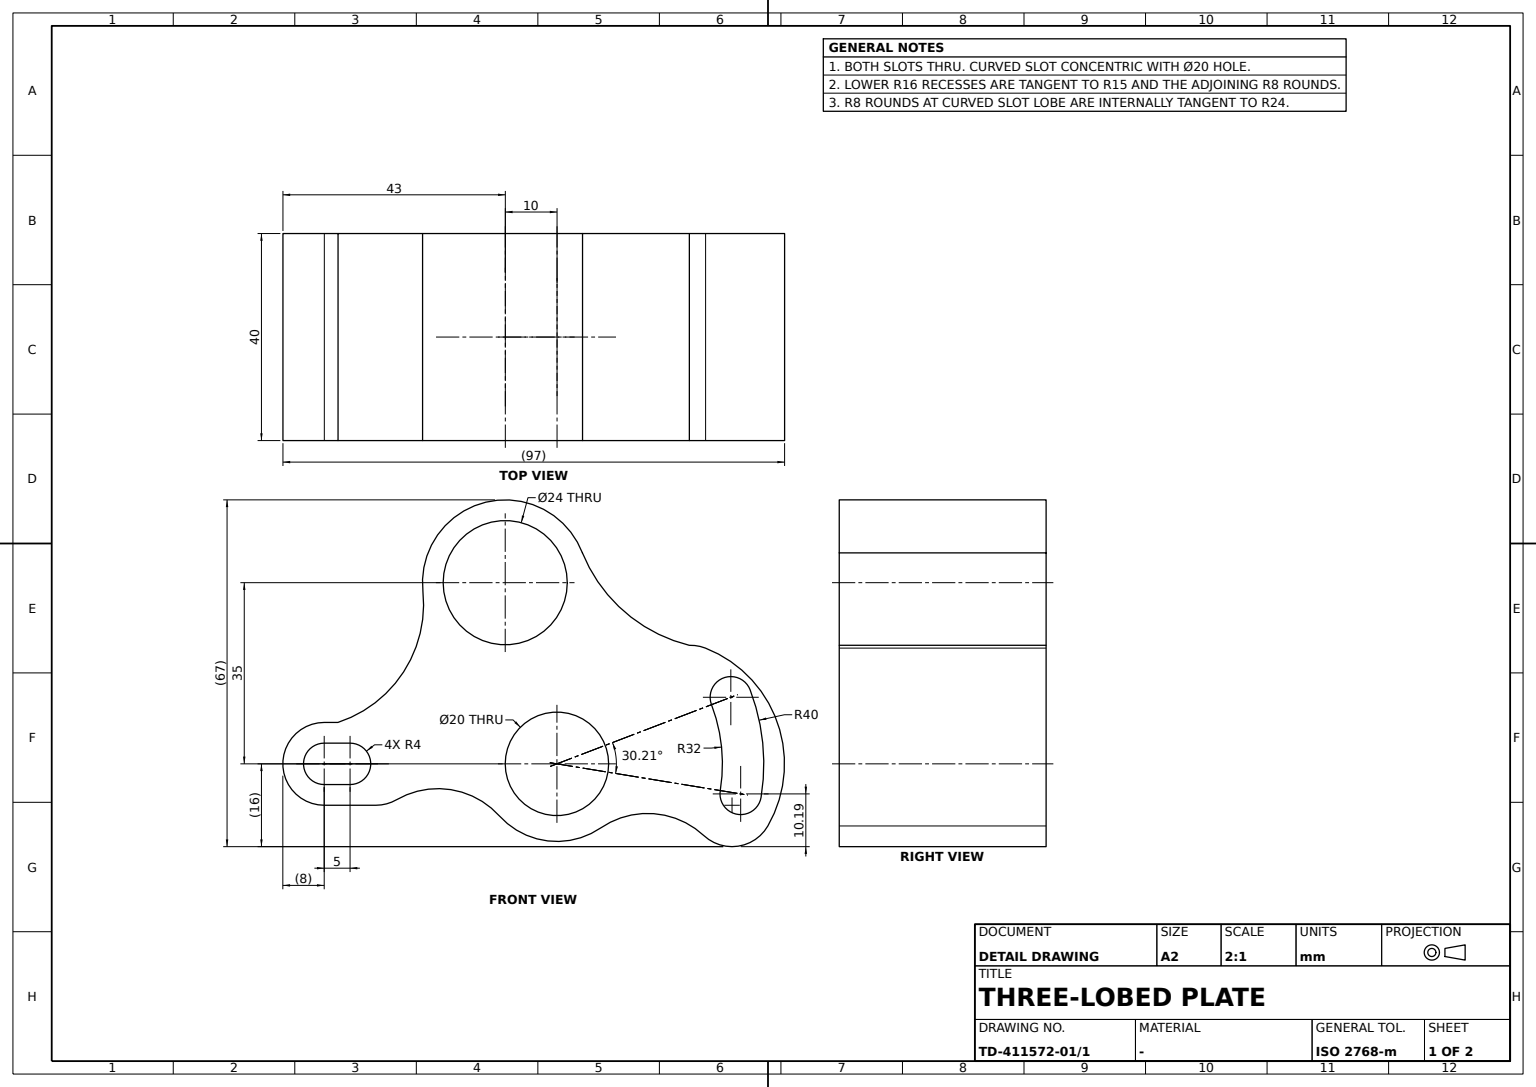
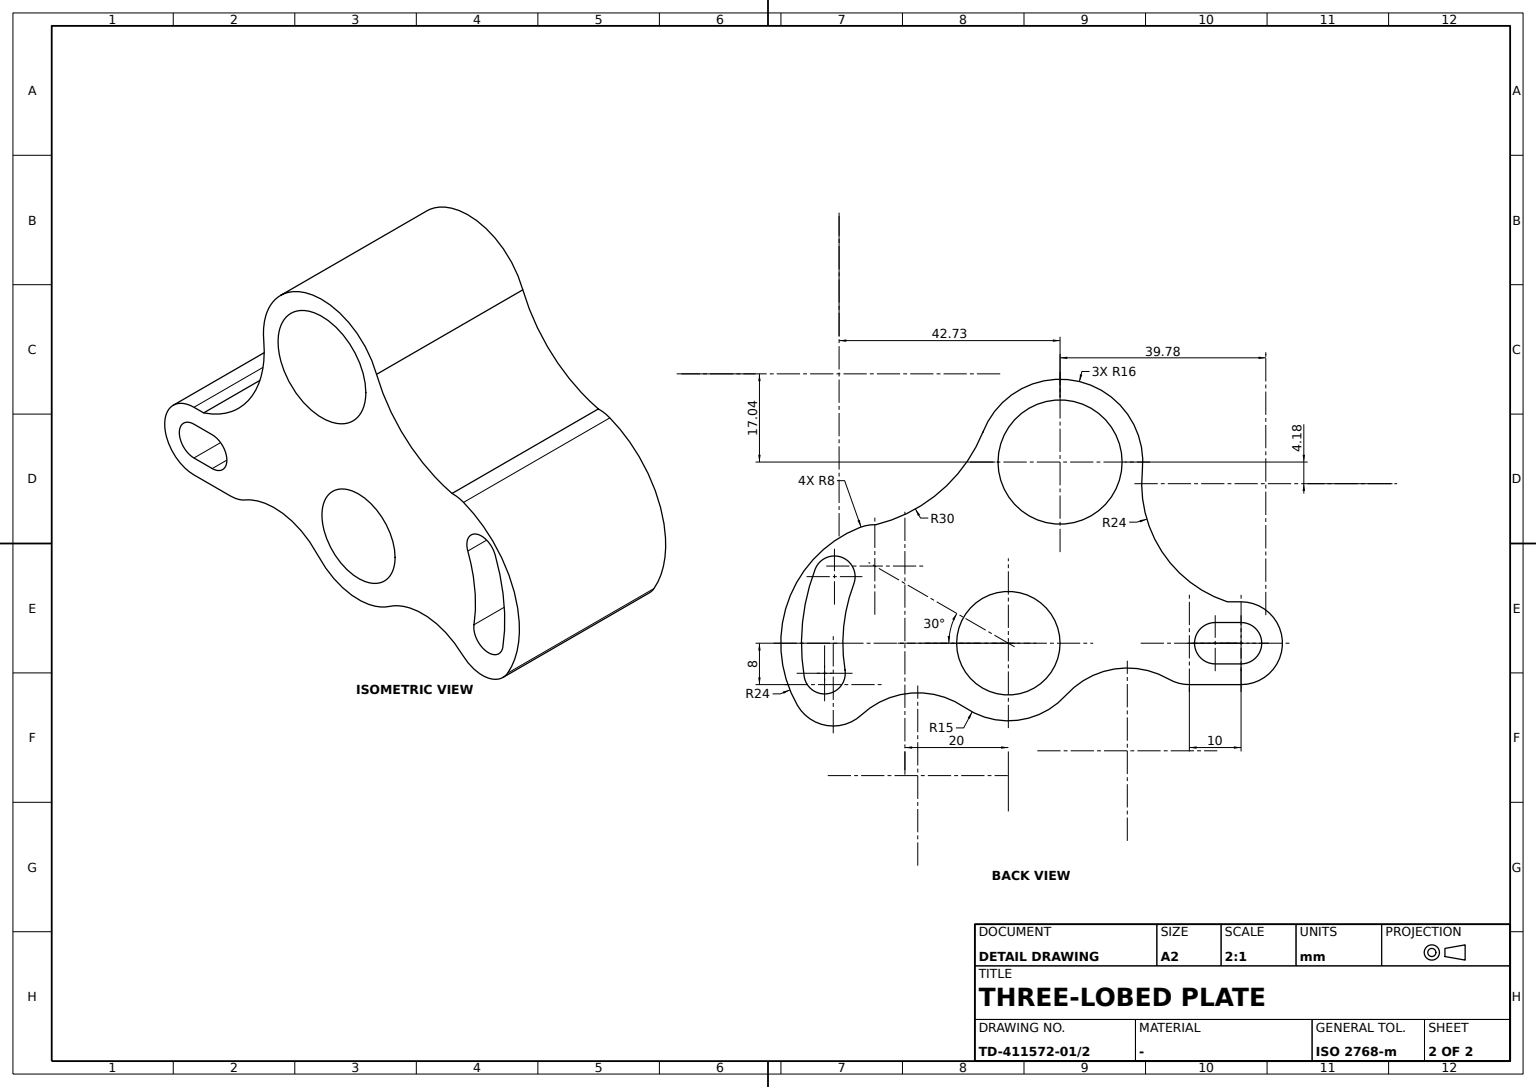
ISO-10303-21;
HEADER;
FILE_DESCRIPTION((''),'2;1');
FILE_NAME('','',(''),(''),'','','');
FILE_SCHEMA(('AUTOMOTIVE_DESIGN'));
ENDSEC;
DATA;
#1=APPLICATION_CONTEXT('');
#2=PRODUCT_CONTEXT('',#1,'mechanical');
#3=PRODUCT('','','',(#2));
#4=PRODUCT_DEFINITION_FORMATION('','',#3);
#5=PRODUCT_DEFINITION_CONTEXT('',#1,'design');
#6=PRODUCT_DEFINITION('','',#4,#5);
#7=PRODUCT_DEFINITION_SHAPE('','',#6);
#8=(LENGTH_UNIT()NAMED_UNIT(*)SI_UNIT(.MILLI.,.METRE.));
#9=(NAMED_UNIT(*)PLANE_ANGLE_UNIT()SI_UNIT($,.RADIAN.));
#10=(NAMED_UNIT(*)SI_UNIT($,.STERADIAN.)SOLID_ANGLE_UNIT());
#11=UNCERTAINTY_MEASURE_WITH_UNIT(LENGTH_MEASURE(0.005),#8,'distance_accuracy_value','');
#12=(GEOMETRIC_REPRESENTATION_CONTEXT(3)GLOBAL_UNCERTAINTY_ASSIGNED_CONTEXT((#11))GLOBAL_UNIT_ASSIGNED_CONTEXT((#8,#9,#10))REPRESENTATION_CONTEXT('',''));
#13=CARTESIAN_POINT('',(47.360506,-20.710402,20.));
#14=VERTEX_POINT('',#13);
#15=CARTESIAN_POINT('',(47.360506,-20.710402,-20.));
#16=VERTEX_POINT('',#15);
#17=CARTESIAN_POINT('',(47.360506,-20.710402,0.));
#18=DIRECTION('',(0.,0.,1.));
#19=VECTOR('',#18,1000.);
#20=LINE('',#17,#19);
#21=EDGE_CURVE('',#14,#16,#20,.F.);
#22=ORIENTED_EDGE('',*,*,#21,.T.);
#23=CARTESIAN_POINT('',(49.47628,-41.451613,-20.));
#24=VERTEX_POINT('',#23);
#25=CARTESIAN_POINT('',(10.,-35.,-20.));
#26=DIRECTION('',(1.,0.,0.));
#27=AXIS2_PLACEMENT_3D('',#25,#18,#26);
#28=CIRCLE('',#27,40.);
#29=EDGE_CURVE('',#24,#16,#28,.T.);
#30=ORIENTED_EDGE('',*,*,#29,.F.);
#31=CARTESIAN_POINT('',(49.47628,-41.451613,20.));
#32=VERTEX_POINT('',#31);
#33=CARTESIAN_POINT('',(49.47628,-41.451613,0.));
#34=LINE('',#33,#19);
#35=EDGE_CURVE('',#32,#24,#34,.F.);
#36=ORIENTED_EDGE('',*,*,#35,.F.);
#37=CARTESIAN_POINT('',(10.,-35.,20.));
#38=AXIS2_PLACEMENT_3D('',#37,#18,#26);
#39=CIRCLE('',#38,40.);
#40=EDGE_CURVE('',#32,#14,#39,.T.);
#41=ORIENTED_EDGE('',*,*,#40,.T.);
#42=EDGE_LOOP('',(#22,#30,#36,#41));
#43=FACE_BOUND('',#42,.T.);
#44=CARTESIAN_POINT('',(10.,-35.,-0.66));
#45=AXIS2_PLACEMENT_3D('',#44,#18,#26);
#46=CYLINDRICAL_SURFACE('',#45,40.);
#47=ADVANCED_FACE('',(#43),#46,.F.);
#48=CARTESIAN_POINT('',(14.92853,5.756648,-20.));
#49=VERTEX_POINT('',#48);
#50=CARTESIAN_POINT('',(14.92853,5.756648,20.));
#51=VERTEX_POINT('',#50);
#52=LINE('',#48,#19);
#53=EDGE_CURVE('',#49,#51,#52,.T.);
#54=ORIENTED_EDGE('',*,*,#53,.F.);
#55=CARTESIAN_POINT('',(-15.91236,-1.672367,-20.));
#56=VERTEX_POINT('',#55);
#57=CARTESIAN_POINT('',(0.,0.,-20.));
#58=AXIS2_PLACEMENT_3D('',#57,#18,#26);
#59=CIRCLE('',#58,16.);
#60=EDGE_CURVE('',#49,#56,#59,.T.);
#61=ORIENTED_EDGE('',*,*,#60,.T.);
#62=CARTESIAN_POINT('',(-15.91236,-1.672367,20.));
#63=VERTEX_POINT('',#62);
#64=CARTESIAN_POINT('',(-15.91236,-1.672367,0.));
#65=LINE('',#64,#19);
#66=EDGE_CURVE('',#56,#63,#65,.T.);
#67=ORIENTED_EDGE('',*,*,#66,.T.);
#68=CARTESIAN_POINT('',(0.,0.,20.));
#69=AXIS2_PLACEMENT_3D('',#68,#18,#26);
#70=CIRCLE('',#69,16.);
#71=EDGE_CURVE('',#51,#63,#70,.T.);
#72=ORIENTED_EDGE('',*,*,#71,.F.);
#73=EDGE_LOOP('',(#54,#61,#67,#72));
#74=FACE_BOUND('',#73,.T.);
#75=CARTESIAN_POINT('',(0.,0.,0.));
#76=AXIS2_PLACEMENT_3D('',#75,#18,#26);
#77=CYLINDRICAL_SURFACE('',#76,16.);
#78=ADVANCED_FACE('',(#74),#77,.T.);
#79=CARTESIAN_POINT('',(39.888404,-23.568321,20.));
#80=VERTEX_POINT('',#79);
#81=CARTESIAN_POINT('',(39.888404,-23.568321,-20.));
#82=VERTEX_POINT('',#81);
#83=CARTESIAN_POINT('',(39.888404,-23.568321,0.));
#84=LINE('',#83,#19);
#85=EDGE_CURVE('',#80,#82,#84,.F.);
#86=ORIENTED_EDGE('',*,*,#85,.F.);
#87=CARTESIAN_POINT('',(41.581024,-40.16129,20.));
#88=VERTEX_POINT('',#87);
#89=CIRCLE('',#38,32.);
#90=EDGE_CURVE('',#88,#80,#89,.T.);
#91=ORIENTED_EDGE('',*,*,#90,.F.);
#92=CARTESIAN_POINT('',(41.581024,-40.16129,-20.));
#93=VERTEX_POINT('',#92);
#94=CARTESIAN_POINT('',(41.581024,-40.16129,0.));
#95=LINE('',#94,#19);
#96=EDGE_CURVE('',#88,#93,#95,.F.);
#97=ORIENTED_EDGE('',*,*,#96,.T.);
#98=CIRCLE('',#27,32.);
#99=EDGE_CURVE('',#93,#82,#98,.T.);
#100=ORIENTED_EDGE('',*,*,#99,.T.);
#101=EDGE_LOOP('',(#86,#91,#97,#100));
#102=FACE_BOUND('',#101,.T.);
#103=CYLINDRICAL_SURFACE('',#45,32.);
#104=ADVANCED_FACE('',(#102),#103,.T.);
#105=ORIENTED_EDGE('',*,*,#96,.F.);
#106=CARTESIAN_POINT('',(45.528652,-40.806452,20.));
#107=AXIS2_PLACEMENT_3D('',#106,#18,#26);
#108=CIRCLE('',#107,4.);
#109=EDGE_CURVE('',#88,#32,#108,.T.);
#110=ORIENTED_EDGE('',*,*,#109,.T.);
#111=ORIENTED_EDGE('',*,*,#35,.T.);
#112=CARTESIAN_POINT('',(45.528652,-40.806452,-20.));
#113=AXIS2_PLACEMENT_3D('',#112,#18,#26);
#114=CIRCLE('',#113,4.);
#115=EDGE_CURVE('',#93,#24,#114,.T.);
#116=ORIENTED_EDGE('',*,*,#115,.F.);
#117=EDGE_LOOP('',(#105,#110,#111,#116));
#118=FACE_BOUND('',#117,.T.);
#119=CARTESIAN_POINT('',(45.528652,-40.806452,-0.66));
#120=AXIS2_PLACEMENT_3D('',#119,#18,#26);
#121=CYLINDRICAL_SURFACE('',#120,4.);
#122=ADVANCED_FACE('',(#118),#121,.F.);
#123=CARTESIAN_POINT('',(38.724981,-12.642122,-20.));
#124=VERTEX_POINT('',#123);
#125=CARTESIAN_POINT('',(35.582075,-12.098188,-20.));
#126=VERTEX_POINT('',#125);
#127=CARTESIAN_POINT('',(35.816654,-20.094748,-20.));
#128=AXIS2_PLACEMENT_3D('',#127,#18,#26);
#129=CIRCLE('',#128,8.);
#130=EDGE_CURVE('',#124,#126,#129,.T.);
#131=ORIENTED_EDGE('',*,*,#130,.T.);
#132=CARTESIAN_POINT('',(35.582075,-12.098188,20.));
#133=VERTEX_POINT('',#132);
#134=LINE('',#125,#19);
#135=EDGE_CURVE('',#126,#133,#134,.T.);
#136=ORIENTED_EDGE('',*,*,#135,.T.);
#137=CARTESIAN_POINT('',(38.724981,-12.642122,20.));
#138=VERTEX_POINT('',#137);
#139=CARTESIAN_POINT('',(35.816654,-20.094748,20.));
#140=AXIS2_PLACEMENT_3D('',#139,#18,#26);
#141=CIRCLE('',#140,8.);
#142=EDGE_CURVE('',#138,#133,#141,.T.);
#143=ORIENTED_EDGE('',*,*,#142,.F.);
#144=CARTESIAN_POINT('',(38.724981,-12.642122,0.));
#145=LINE('',#144,#19);
#146=EDGE_CURVE('',#124,#138,#145,.T.);
#147=ORIENTED_EDGE('',*,*,#146,.F.);
#148=EDGE_LOOP('',(#131,#136,#143,#147));
#149=FACE_BOUND('',#148,.T.);
#150=CARTESIAN_POINT('',(35.816654,-20.094748,0.));
#151=AXIS2_PLACEMENT_3D('',#150,#18,#26);
#152=CYLINDRICAL_SURFACE('',#151,8.);
#153=ADVANCED_FACE('',(#149),#152,.T.);
#154=ORIENTED_EDGE('',*,*,#146,.T.);
#155=CARTESIAN_POINT('',(50.78461,-47.,20.));
#156=VERTEX_POINT('',#155);
#157=CARTESIAN_POINT('',(30.,-35.,20.));
#158=AXIS2_PLACEMENT_3D('',#157,#18,#26);
#159=CIRCLE('',#158,24.);
#160=EDGE_CURVE('',#156,#138,#159,.T.);
#161=ORIENTED_EDGE('',*,*,#160,.F.);
#162=CARTESIAN_POINT('',(50.78461,-47.,-20.));
#163=VERTEX_POINT('',#162);
#164=CARTESIAN_POINT('',(50.78461,-47.,0.));
#165=LINE('',#164,#19);
#166=EDGE_CURVE('',#163,#156,#165,.T.);
#167=ORIENTED_EDGE('',*,*,#166,.F.);
#168=CARTESIAN_POINT('',(30.,-35.,-20.));
#169=AXIS2_PLACEMENT_3D('',#168,#18,#26);
#170=CIRCLE('',#169,24.);
#171=EDGE_CURVE('',#163,#124,#170,.T.);
#172=ORIENTED_EDGE('',*,*,#171,.T.);
#173=EDGE_LOOP('',(#154,#161,#167,#172));
#174=FACE_BOUND('',#173,.T.);
#175=CARTESIAN_POINT('',(30.,-35.,0.));
#176=AXIS2_PLACEMENT_3D('',#175,#18,#26);
#177=CYLINDRICAL_SURFACE('',#176,24.);
#178=ADVANCED_FACE('',(#174),#177,.T.);
#179=CARTESIAN_POINT('',(-35.,-31.,20.));
#180=VERTEX_POINT('',#179);
#181=CARTESIAN_POINT('',(-30.,-31.,20.));
#182=VERTEX_POINT('',#181);
#183=VECTOR('',#26,1000.);
#184=LINE('',#179,#183);
#185=EDGE_CURVE('',#180,#182,#184,.T.);
#186=ORIENTED_EDGE('',*,*,#185,.F.);
#187=CARTESIAN_POINT('',(-35.,-31.,-20.));
#188=VERTEX_POINT('',#187);
#189=CARTESIAN_POINT('',(-35.,-31.,-0.66));
#190=LINE('',#189,#19);
#191=EDGE_CURVE('',#180,#188,#190,.F.);
#192=ORIENTED_EDGE('',*,*,#191,.T.);
#193=CARTESIAN_POINT('',(-30.,-31.,-20.));
#194=VERTEX_POINT('',#193);
#195=LINE('',#187,#183);
#196=EDGE_CURVE('',#188,#194,#195,.T.);
#197=ORIENTED_EDGE('',*,*,#196,.T.);
#198=CARTESIAN_POINT('',(-30.,-31.,-0.66));
#199=LINE('',#198,#19);
#200=EDGE_CURVE('',#182,#194,#199,.F.);
#201=ORIENTED_EDGE('',*,*,#200,.F.);
#202=EDGE_LOOP('',(#186,#192,#197,#201));
#203=FACE_BOUND('',#202,.T.);
#204=DIRECTION('',(0.,1.,0.));
#205=AXIS2_PLACEMENT_3D('',#179,#204,#26);
#206=PLANE('',#205);
#207=ADVANCED_FACE('',(#203),#206,.F.);
#208=CARTESIAN_POINT('',(-35.,-39.,20.));
#209=VERTEX_POINT('',#208);
#210=CARTESIAN_POINT('',(-35.,-35.,20.));
#211=AXIS2_PLACEMENT_3D('',#210,#18,#26);
#212=CIRCLE('',#211,4.);
#213=EDGE_CURVE('',#180,#209,#212,.T.);
#214=ORIENTED_EDGE('',*,*,#213,.T.);
#215=CARTESIAN_POINT('',(-35.,-39.,-20.));
#216=VERTEX_POINT('',#215);
#217=CARTESIAN_POINT('',(-35.,-39.,-0.66));
#218=LINE('',#217,#19);
#219=EDGE_CURVE('',#209,#216,#218,.F.);
#220=ORIENTED_EDGE('',*,*,#219,.T.);
#221=CARTESIAN_POINT('',(-35.,-35.,-20.));
#222=AXIS2_PLACEMENT_3D('',#221,#18,#26);
#223=CIRCLE('',#222,4.);
#224=EDGE_CURVE('',#188,#216,#223,.T.);
#225=ORIENTED_EDGE('',*,*,#224,.F.);
#226=ORIENTED_EDGE('',*,*,#191,.F.);
#227=EDGE_LOOP('',(#214,#220,#225,#226));
#228=FACE_BOUND('',#227,.T.);
#229=CARTESIAN_POINT('',(-35.,-35.,-0.66));
#230=AXIS2_PLACEMENT_3D('',#229,#18,#26);
#231=CYLINDRICAL_SURFACE('',#230,4.);
#232=ADVANCED_FACE('',(#228),#231,.F.);
#233=CARTESIAN_POINT('',(-25.,-43.,-20.));
#234=VERTEX_POINT('',#233);
#235=CARTESIAN_POINT('',(-25.,-43.,20.));
#236=VERTEX_POINT('',#235);
#237=CARTESIAN_POINT('',(-25.,-43.,0.));
#238=LINE('',#237,#19);
#239=EDGE_CURVE('',#234,#236,#238,.T.);
#240=ORIENTED_EDGE('',*,*,#239,.F.);
#241=CARTESIAN_POINT('',(-21.,-41.928203,-20.));
#242=VERTEX_POINT('',#241);
#243=CARTESIAN_POINT('',(-25.,-35.,-20.));
#244=AXIS2_PLACEMENT_3D('',#243,#18,#26);
#245=CIRCLE('',#244,8.);
#246=EDGE_CURVE('',#234,#242,#245,.T.);
#247=ORIENTED_EDGE('',*,*,#246,.T.);
#248=CARTESIAN_POINT('',(-21.,-41.928203,20.));
#249=VERTEX_POINT('',#248);
#250=CARTESIAN_POINT('',(-21.,-41.928203,0.));
#251=LINE('',#250,#19);
#252=EDGE_CURVE('',#242,#249,#251,.T.);
#253=ORIENTED_EDGE('',*,*,#252,.T.);
#254=CARTESIAN_POINT('',(-25.,-35.,20.));
#255=AXIS2_PLACEMENT_3D('',#254,#18,#26);
#256=CIRCLE('',#255,8.);
#257=EDGE_CURVE('',#236,#249,#256,.T.);
#258=ORIENTED_EDGE('',*,*,#257,.F.);
#259=EDGE_LOOP('',(#240,#247,#253,#258));
#260=FACE_BOUND('',#259,.T.);
#261=CARTESIAN_POINT('',(-25.,-35.,0.));
#262=AXIS2_PLACEMENT_3D('',#261,#18,#26);
#263=CYLINDRICAL_SURFACE('',#262,8.);
#264=ADVANCED_FACE('',(#260),#263,.T.);
#265=CARTESIAN_POINT('',(-30.,-39.,20.));
#266=VERTEX_POINT('',#265);
#267=CARTESIAN_POINT('',(-30.,-35.,20.));
#268=AXIS2_PLACEMENT_3D('',#267,#18,#26);
#269=CIRCLE('',#268,4.);
#270=EDGE_CURVE('',#266,#182,#269,.T.);
#271=ORIENTED_EDGE('',*,*,#270,.T.);
#272=ORIENTED_EDGE('',*,*,#200,.T.);
#273=CARTESIAN_POINT('',(-30.,-39.,-20.));
#274=VERTEX_POINT('',#273);
#275=CARTESIAN_POINT('',(-30.,-35.,-20.));
#276=AXIS2_PLACEMENT_3D('',#275,#18,#26);
#277=CIRCLE('',#276,4.);
#278=EDGE_CURVE('',#274,#194,#277,.T.);
#279=ORIENTED_EDGE('',*,*,#278,.F.);
#280=CARTESIAN_POINT('',(-30.,-39.,-0.66));
#281=LINE('',#280,#19);
#282=EDGE_CURVE('',#266,#274,#281,.F.);
#283=ORIENTED_EDGE('',*,*,#282,.F.);
#284=EDGE_LOOP('',(#271,#272,#279,#283));
#285=FACE_BOUND('',#284,.T.);
#286=CARTESIAN_POINT('',(-30.,-35.,-0.66));
#287=AXIS2_PLACEMENT_3D('',#286,#18,#26);
#288=CYLINDRICAL_SURFACE('',#287,4.);
#289=ADVANCED_FACE('',(#285),#288,.F.);
#290=CARTESIAN_POINT('',(-35.,-27.,20.));
#291=VERTEX_POINT('',#290);
#292=CARTESIAN_POINT('',(-32.345209,-27.,20.));
#293=VERTEX_POINT('',#292);
#294=CARTESIAN_POINT('',(0.,-27.,20.));
#295=LINE('',#294,#183);
#296=EDGE_CURVE('',#291,#293,#295,.T.);
#297=ORIENTED_EDGE('',*,*,#296,.T.);
#298=CARTESIAN_POINT('',(-32.345209,-27.,-20.));
#299=VERTEX_POINT('',#298);
#300=LINE('',#298,#19);
#301=EDGE_CURVE('',#299,#293,#300,.T.);
#302=ORIENTED_EDGE('',*,*,#301,.F.);
#303=CARTESIAN_POINT('',(-35.,-27.,-20.));
#304=VERTEX_POINT('',#303);
#305=CARTESIAN_POINT('',(0.,-27.,-20.));
#306=LINE('',#305,#183);
#307=EDGE_CURVE('',#304,#299,#306,.T.);
#308=ORIENTED_EDGE('',*,*,#307,.F.);
#309=CARTESIAN_POINT('',(-35.,-27.,0.));
#310=LINE('',#309,#19);
#311=EDGE_CURVE('',#304,#291,#310,.T.);
#312=ORIENTED_EDGE('',*,*,#311,.T.);
#313=EDGE_LOOP('',(#297,#302,#308,#312));
#314=FACE_BOUND('',#313,.T.);
#315=DIRECTION('',(0.,-1.,0.));
#316=AXIS2_PLACEMENT_3D('',#309,#315,#26);
#317=PLANE('',#316);
#318=ADVANCED_FACE('',(#314),#317,.F.);
#319=CARTESIAN_POINT('',(18.475181,-47.376239,-20.));
#320=VERTEX_POINT('',#319);
#321=CARTESIAN_POINT('',(18.475181,-47.376239,20.));
#322=VERTEX_POINT('',#321);
#323=CARTESIAN_POINT('',(18.475181,-47.376239,0.));
#324=LINE('',#323,#19);
#325=EDGE_CURVE('',#320,#322,#324,.T.);
#326=ORIENTED_EDGE('',*,*,#325,.T.);
#327=CARTESIAN_POINT('',(-1.129032,-45.057069,20.));
#328=VERTEX_POINT('',#327);
#329=CIRCLE('',#38,15.);
#330=EDGE_CURVE('',#328,#322,#329,.T.);
#331=ORIENTED_EDGE('',*,*,#330,.F.);
#332=CARTESIAN_POINT('',(-1.129032,-45.057069,-20.));
#333=VERTEX_POINT('',#332);
#334=CARTESIAN_POINT('',(-1.129032,-45.057069,0.));
#335=LINE('',#334,#19);
#336=EDGE_CURVE('',#333,#328,#335,.T.);
#337=ORIENTED_EDGE('',*,*,#336,.F.);
#338=CIRCLE('',#27,15.);
#339=EDGE_CURVE('',#333,#320,#338,.T.);
#340=ORIENTED_EDGE('',*,*,#339,.T.);
#341=EDGE_LOOP('',(#326,#331,#337,#340));
#342=FACE_BOUND('',#341,.T.);
#343=CARTESIAN_POINT('',(10.,-35.,0.));
#344=AXIS2_PLACEMENT_3D('',#343,#18,#26);
#345=CYLINDRICAL_SURFACE('',#344,15.);
#346=ADVANCED_FACE('',(#342),#345,.T.);
#347=ORIENTED_EDGE('',*,*,#325,.F.);
#348=CARTESIAN_POINT('',(38.409396,-48.859187,-20.));
#349=VERTEX_POINT('',#348);
#350=CARTESIAN_POINT('',(27.515374,-60.577562,-20.));
#351=AXIS2_PLACEMENT_3D('',#350,#18,#26);
#352=CIRCLE('',#351,16.);
#353=EDGE_CURVE('',#349,#320,#352,.T.);
#354=ORIENTED_EDGE('',*,*,#353,.F.);
#355=CARTESIAN_POINT('',(38.409396,-48.859187,20.));
#356=VERTEX_POINT('',#355);
#357=CARTESIAN_POINT('',(38.409396,-48.859187,0.));
#358=LINE('',#357,#19);
#359=EDGE_CURVE('',#349,#356,#358,.T.);
#360=ORIENTED_EDGE('',*,*,#359,.T.);
#361=CARTESIAN_POINT('',(27.515374,-60.577562,20.));
#362=AXIS2_PLACEMENT_3D('',#361,#18,#26);
#363=CIRCLE('',#362,16.);
#364=EDGE_CURVE('',#356,#322,#363,.T.);
#365=ORIENTED_EDGE('',*,*,#364,.T.);
#366=EDGE_LOOP('',(#347,#354,#360,#365));
#367=FACE_BOUND('',#366,.T.);
#368=CARTESIAN_POINT('',(27.515374,-60.577562,0.));
#369=AXIS2_PLACEMENT_3D('',#368,#18,#26);
#370=CYLINDRICAL_SURFACE('',#369,16.);
#371=ADVANCED_FACE('',(#367),#370,.F.);
#372=ORIENTED_EDGE('',*,*,#166,.T.);
#373=CARTESIAN_POINT('',(43.856406,-43.,20.));
#374=AXIS2_PLACEMENT_3D('',#373,#18,#26);
#375=CIRCLE('',#374,8.);
#376=EDGE_CURVE('',#356,#156,#375,.T.);
#377=ORIENTED_EDGE('',*,*,#376,.F.);
#378=ORIENTED_EDGE('',*,*,#359,.F.);
#379=CARTESIAN_POINT('',(43.856406,-43.,-20.));
#380=AXIS2_PLACEMENT_3D('',#379,#18,#26);
#381=CIRCLE('',#380,8.);
#382=EDGE_CURVE('',#349,#163,#381,.T.);
#383=ORIENTED_EDGE('',*,*,#382,.T.);
#384=EDGE_LOOP('',(#372,#377,#378,#383));
#385=FACE_BOUND('',#384,.T.);
#386=CARTESIAN_POINT('',(43.856406,-43.,0.));
#387=AXIS2_PLACEMENT_3D('',#386,#18,#26);
#388=CYLINDRICAL_SURFACE('',#387,8.);
#389=ADVANCED_FACE('',(#385),#388,.T.);
#390=ORIENTED_EDGE('',*,*,#336,.T.);
#391=CARTESIAN_POINT('',(-13.,-55.78461,20.));
#392=AXIS2_PLACEMENT_3D('',#391,#18,#26);
#393=CIRCLE('',#392,16.);
#394=EDGE_CURVE('',#328,#249,#393,.T.);
#395=ORIENTED_EDGE('',*,*,#394,.T.);
#396=ORIENTED_EDGE('',*,*,#252,.F.);
#397=CARTESIAN_POINT('',(-13.,-55.78461,-20.));
#398=AXIS2_PLACEMENT_3D('',#397,#18,#26);
#399=CIRCLE('',#398,16.);
#400=EDGE_CURVE('',#333,#242,#399,.T.);
#401=ORIENTED_EDGE('',*,*,#400,.F.);
#402=EDGE_LOOP('',(#390,#395,#396,#401));
#403=FACE_BOUND('',#402,.T.);
#404=CARTESIAN_POINT('',(-13.,-55.78461,0.));
#405=AXIS2_PLACEMENT_3D('',#404,#18,#26);
#406=CYLINDRICAL_SURFACE('',#405,16.);
#407=ADVANCED_FACE('',(#403),#406,.F.);
#408=DIRECTION('',(-1.,0.,0.));
#409=VECTOR('',#408,1000.);
#410=LINE('',#265,#409);
#411=EDGE_CURVE('',#266,#209,#410,.T.);
#412=ORIENTED_EDGE('',*,*,#411,.F.);
#413=ORIENTED_EDGE('',*,*,#282,.T.);
#414=LINE('',#273,#409);
#415=EDGE_CURVE('',#274,#216,#414,.T.);
#416=ORIENTED_EDGE('',*,*,#415,.T.);
#417=ORIENTED_EDGE('',*,*,#219,.F.);
#418=EDGE_LOOP('',(#412,#413,#416,#417));
#419=FACE_BOUND('',#418,.T.);
#420=AXIS2_PLACEMENT_3D('',#265,#315,#408);
#421=PLANE('',#420);
#422=ADVANCED_FACE('',(#419),#421,.F.);
#423=CARTESIAN_POINT('',(20.,-35.,-20.));
#424=VERTEX_POINT('',#423);
#425=CIRCLE('',#27,10.);
#426=EDGE_CURVE('',#424,#424,#425,.T.);
#427=ORIENTED_EDGE('',*,*,#426,.T.);
#428=EDGE_LOOP('',(#427));
#429=FACE_BOUND('',#428,.T.);
#430=CARTESIAN_POINT('',(12.,0.,-20.));
#431=VERTEX_POINT('',#430);
#432=CIRCLE('',#58,12.);
#433=EDGE_CURVE('',#431,#431,#432,.T.);
#434=ORIENTED_EDGE('',*,*,#433,.T.);
#435=EDGE_LOOP('',(#434));
#436=FACE_BOUND('',#435,.T.);
#437=ORIENTED_EDGE('',*,*,#278,.T.);
#438=ORIENTED_EDGE('',*,*,#196,.F.);
#439=ORIENTED_EDGE('',*,*,#224,.T.);
#440=ORIENTED_EDGE('',*,*,#415,.F.);
#441=EDGE_LOOP('',(#437,#438,#439,#440));
#442=FACE_BOUND('',#441,.T.);
#443=ORIENTED_EDGE('',*,*,#339,.F.);
#444=ORIENTED_EDGE('',*,*,#400,.T.);
#445=ORIENTED_EDGE('',*,*,#246,.F.);
#446=CARTESIAN_POINT('',(-35.,-43.,-20.));
#447=VERTEX_POINT('',#446);
#448=CARTESIAN_POINT('',(0.,-43.,-20.));
#449=LINE('',#448,#409);
#450=EDGE_CURVE('',#234,#447,#449,.T.);
#451=ORIENTED_EDGE('',*,*,#450,.T.);
#452=CIRCLE('',#222,8.);
#453=EDGE_CURVE('',#304,#447,#452,.T.);
#454=ORIENTED_EDGE('',*,*,#453,.F.);
#455=ORIENTED_EDGE('',*,*,#307,.T.);
#456=CARTESIAN_POINT('',(-39.780899,-4.180918,-20.));
#457=AXIS2_PLACEMENT_3D('',#456,#18,#26);
#458=CIRCLE('',#457,24.);
#459=EDGE_CURVE('',#299,#56,#458,.T.);
#460=ORIENTED_EDGE('',*,*,#459,.T.);
#461=ORIENTED_EDGE('',*,*,#60,.F.);
#462=CARTESIAN_POINT('',(42.726272,17.038738,-20.));
#463=AXIS2_PLACEMENT_3D('',#462,#18,#26);
#464=CIRCLE('',#463,30.);
#465=EDGE_CURVE('',#49,#126,#464,.T.);
#466=ORIENTED_EDGE('',*,*,#465,.T.);
#467=ORIENTED_EDGE('',*,*,#130,.F.);
#468=ORIENTED_EDGE('',*,*,#171,.F.);
#469=ORIENTED_EDGE('',*,*,#382,.F.);
#470=ORIENTED_EDGE('',*,*,#353,.T.);
#471=EDGE_LOOP('',(#443,#444,#445,#451,#454,#455,#460,#461,#466,#467,#468,#469,#470));
#472=FACE_BOUND('',#471,.T.);
#473=ORIENTED_EDGE('',*,*,#115,.T.);
#474=ORIENTED_EDGE('',*,*,#29,.T.);
#475=CARTESIAN_POINT('',(43.624455,-22.139362,-20.));
#476=AXIS2_PLACEMENT_3D('',#475,#18,#26);
#477=CIRCLE('',#476,4.);
#478=EDGE_CURVE('',#16,#82,#477,.T.);
#479=ORIENTED_EDGE('',*,*,#478,.T.);
#480=ORIENTED_EDGE('',*,*,#99,.F.);
#481=EDGE_LOOP('',(#473,#474,#479,#480));
#482=FACE_BOUND('',#481,.T.);
#483=PLANE('',#58);
#484=ADVANCED_FACE('',(#429,#436,#442,#472,#482),#483,.F.);
#485=CARTESIAN_POINT('',(20.,-35.,20.));
#486=VERTEX_POINT('',#485);
#487=CIRCLE('',#38,10.);
#488=EDGE_CURVE('',#486,#486,#487,.T.);
#489=ORIENTED_EDGE('',*,*,#488,.T.);
#490=EDGE_LOOP('',(#489));
#491=FACE_BOUND('',#490,.T.);
#492=ORIENTED_EDGE('',*,*,#426,.F.);
#493=EDGE_LOOP('',(#492));
#494=FACE_BOUND('',#493,.T.);
#495=CYLINDRICAL_SURFACE('',#45,10.);
#496=ADVANCED_FACE('',(#491,#494),#495,.F.);
#497=CARTESIAN_POINT('',(-35.,-43.,20.));
#498=VERTEX_POINT('',#497);
#499=CARTESIAN_POINT('',(0.,-43.,20.));
#500=LINE('',#499,#409);
#501=EDGE_CURVE('',#236,#498,#500,.T.);
#502=ORIENTED_EDGE('',*,*,#501,.T.);
#503=CARTESIAN_POINT('',(-35.,-43.,0.));
#504=LINE('',#503,#19);
#505=EDGE_CURVE('',#447,#498,#504,.T.);
#506=ORIENTED_EDGE('',*,*,#505,.F.);
#507=ORIENTED_EDGE('',*,*,#450,.F.);
#508=ORIENTED_EDGE('',*,*,#239,.T.);
#509=EDGE_LOOP('',(#502,#506,#507,#508));
#510=FACE_BOUND('',#509,.T.);
#511=AXIS2_PLACEMENT_3D('',#237,#204,#408);
#512=PLANE('',#511);
#513=ADVANCED_FACE('',(#510),#512,.F.);
#514=CARTESIAN_POINT('',(12.,0.,20.));
#515=VERTEX_POINT('',#514);
#516=CIRCLE('',#69,12.);
#517=EDGE_CURVE('',#515,#515,#516,.T.);
#518=ORIENTED_EDGE('',*,*,#517,.F.);
#519=EDGE_LOOP('',(#518));
#520=FACE_BOUND('',#519,.T.);
#521=CARTESIAN_POINT('',(42.726272,17.038738,20.));
#522=AXIS2_PLACEMENT_3D('',#521,#18,#26);
#523=CIRCLE('',#522,30.);
#524=EDGE_CURVE('',#51,#133,#523,.T.);
#525=ORIENTED_EDGE('',*,*,#524,.F.);
#526=ORIENTED_EDGE('',*,*,#71,.T.);
#527=CARTESIAN_POINT('',(-39.780899,-4.180918,20.));
#528=AXIS2_PLACEMENT_3D('',#527,#18,#26);
#529=CIRCLE('',#528,24.);
#530=EDGE_CURVE('',#293,#63,#529,.T.);
#531=ORIENTED_EDGE('',*,*,#530,.F.);
#532=ORIENTED_EDGE('',*,*,#296,.F.);
#533=CIRCLE('',#211,8.);
#534=EDGE_CURVE('',#291,#498,#533,.T.);
#535=ORIENTED_EDGE('',*,*,#534,.T.);
#536=ORIENTED_EDGE('',*,*,#501,.F.);
#537=ORIENTED_EDGE('',*,*,#257,.T.);
#538=ORIENTED_EDGE('',*,*,#394,.F.);
#539=ORIENTED_EDGE('',*,*,#330,.T.);
#540=ORIENTED_EDGE('',*,*,#364,.F.);
#541=ORIENTED_EDGE('',*,*,#376,.T.);
#542=ORIENTED_EDGE('',*,*,#160,.T.);
#543=ORIENTED_EDGE('',*,*,#142,.T.);
#544=EDGE_LOOP('',(#525,#526,#531,#532,#535,#536,#537,#538,#539,#540,#541,#542,#543));
#545=FACE_BOUND('',#544,.T.);
#546=ORIENTED_EDGE('',*,*,#40,.F.);
#547=ORIENTED_EDGE('',*,*,#109,.F.);
#548=ORIENTED_EDGE('',*,*,#90,.T.);
#549=CARTESIAN_POINT('',(43.624455,-22.139362,20.));
#550=AXIS2_PLACEMENT_3D('',#549,#18,#26);
#551=CIRCLE('',#550,4.);
#552=EDGE_CURVE('',#14,#80,#551,.T.);
#553=ORIENTED_EDGE('',*,*,#552,.F.);
#554=EDGE_LOOP('',(#546,#547,#548,#553));
#555=FACE_BOUND('',#554,.T.);
#556=ORIENTED_EDGE('',*,*,#411,.T.);
#557=ORIENTED_EDGE('',*,*,#213,.F.);
#558=ORIENTED_EDGE('',*,*,#185,.T.);
#559=ORIENTED_EDGE('',*,*,#270,.F.);
#560=EDGE_LOOP('',(#556,#557,#558,#559));
#561=FACE_BOUND('',#560,.T.);
#562=ORIENTED_EDGE('',*,*,#488,.F.);
#563=EDGE_LOOP('',(#562));
#564=FACE_BOUND('',#563,.T.);
#565=PLANE('',#69);
#566=ADVANCED_FACE('',(#520,#545,#555,#561,#564),#565,.T.);
#567=ORIENTED_EDGE('',*,*,#478,.F.);
#568=ORIENTED_EDGE('',*,*,#21,.F.);
#569=ORIENTED_EDGE('',*,*,#552,.T.);
#570=ORIENTED_EDGE('',*,*,#85,.T.);
#571=EDGE_LOOP('',(#567,#568,#569,#570));
#572=FACE_BOUND('',#571,.T.);
#573=CARTESIAN_POINT('',(43.624455,-22.139362,-0.66));
#574=AXIS2_PLACEMENT_3D('',#573,#18,#26);
#575=CYLINDRICAL_SURFACE('',#574,4.);
#576=ADVANCED_FACE('',(#572),#575,.F.);
#577=ORIENTED_EDGE('',*,*,#517,.T.);
#578=EDGE_LOOP('',(#577));
#579=FACE_BOUND('',#578,.T.);
#580=ORIENTED_EDGE('',*,*,#433,.F.);
#581=EDGE_LOOP('',(#580));
#582=FACE_BOUND('',#581,.T.);
#583=CARTESIAN_POINT('',(0.,0.,-0.66));
#584=AXIS2_PLACEMENT_3D('',#583,#18,#26);
#585=CYLINDRICAL_SURFACE('',#584,12.);
#586=ADVANCED_FACE('',(#579,#582),#585,.F.);
#587=ORIENTED_EDGE('',*,*,#301,.T.);
#588=ORIENTED_EDGE('',*,*,#530,.T.);
#589=ORIENTED_EDGE('',*,*,#66,.F.);
#590=ORIENTED_EDGE('',*,*,#459,.F.);
#591=EDGE_LOOP('',(#587,#588,#589,#590));
#592=FACE_BOUND('',#591,.T.);
#593=CARTESIAN_POINT('',(-39.780899,-4.180918,0.));
#594=AXIS2_PLACEMENT_3D('',#593,#18,#26);
#595=CYLINDRICAL_SURFACE('',#594,24.);
#596=ADVANCED_FACE('',(#592),#595,.F.);
#597=ORIENTED_EDGE('',*,*,#505,.T.);
#598=ORIENTED_EDGE('',*,*,#534,.F.);
#599=ORIENTED_EDGE('',*,*,#311,.F.);
#600=ORIENTED_EDGE('',*,*,#453,.T.);
#601=EDGE_LOOP('',(#597,#598,#599,#600));
#602=FACE_BOUND('',#601,.T.);
#603=CARTESIAN_POINT('',(-35.,-35.,0.));
#604=AXIS2_PLACEMENT_3D('',#603,#18,#26);
#605=CYLINDRICAL_SURFACE('',#604,8.);
#606=ADVANCED_FACE('',(#602),#605,.T.);
#607=ORIENTED_EDGE('',*,*,#524,.T.);
#608=ORIENTED_EDGE('',*,*,#135,.F.);
#609=ORIENTED_EDGE('',*,*,#465,.F.);
#610=ORIENTED_EDGE('',*,*,#53,.T.);
#611=EDGE_LOOP('',(#607,#608,#609,#610));
#612=FACE_BOUND('',#611,.T.);
#613=CARTESIAN_POINT('',(42.726272,17.038738,0.));
#614=AXIS2_PLACEMENT_3D('',#613,#18,#26);
#615=CYLINDRICAL_SURFACE('',#614,30.);
#616=ADVANCED_FACE('',(#612),#615,.F.);
#617=CLOSED_SHELL('',(#47,#78,#104,#122,#153,#178,#207,#232,#264,#289,#318,#346,#371,#389,#407,#422,#484,#496,#513,#566,#576,#586,#596,#606,#616));
#618=MANIFOLD_SOLID_BREP('',#617);
#619=ADVANCED_BREP_SHAPE_REPRESENTATION('',(#618),#12);
#620=SHAPE_DEFINITION_REPRESENTATION(#7,#619);
ENDSEC;
END-ISO-10303-21;
